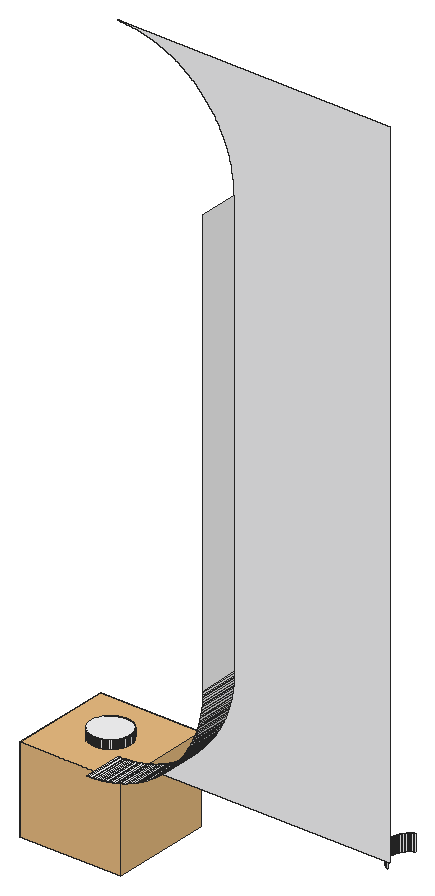
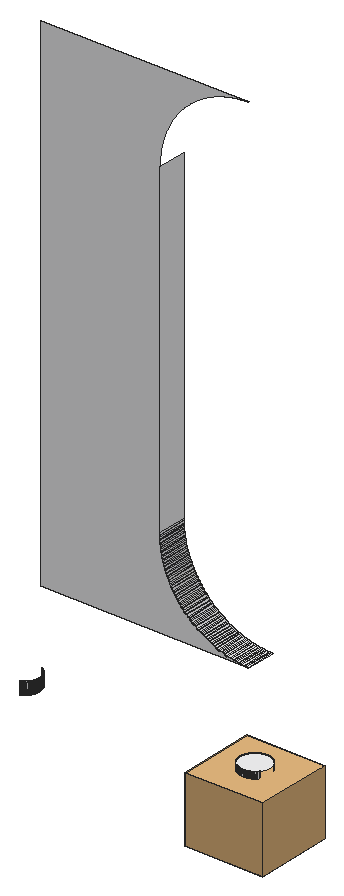
# SketchUp Ruby script. Lengths in inches.
U = 1.inch
M = Sketchup.active_model
def pt(a) = Geom::Point3d.new(a.map { |v| v * U })
def face(e, loops, mat)
  f = e.add_face(loops[0].map { |a| pt(a) })
  loops[1..].each { |l| e.add_face(l.map { |a| pt(a) }).erase! }
  f.material = f.back_material = mat if mat
  f
end
# faces: each face lists its corners as indices into pts; further lists are holes
def faces(e, pts, list, mat = nil) = list.each { |f| face(e, (f[0].is_a?(Array) ? f : [f]).map { |l| l.map { |i| pts[i] } }, mat) }
# xy, xz, yz: faces in a plane at the given z, y or x. An outline is a flat list of corners, or four numbers for a rectangle; further outlines are holes
def ring(l) = l.size == 4 ? [[l[0], l[1]], [l[2], l[1]], [l[2], l[3]], [l[0], l[3]]] : l.each_slice(2).to_a
def flat(e, list, mat, &to3) = list.each { |f| face(e, (f[0].is_a?(Array) ? f : [f]).map { |l| ring(l).map { |u, v| to3.(u, v) } }, mat) }
def xy(e, z, list, mat = nil) = flat(e, list, mat) { |x, y| [x, y, z] }
def xz(e, y, list, mat = nil) = flat(e, list, mat) { |x, z| [x, y, z] }
def yz(e, x, list, mat = nil) = flat(e, list, mat) { |y, z| [x, y, z] }
def lines(e, pts, list) = list.each { |a, b| e.add_line(pt(pts[a]), pt(pts[b])) }
# prism: a flat outline (further loops are holes) pulled along v
def prism(e, loops, v, mat = nil)
  f = face(e, loops, mat); d = Geom::Vector3d.new(v.map { |x| x * U })
  f.pushpull(f.normal.samedirection?(d) ? d.length : -d.length)
end
def box(e, o, s, mat = nil) = prism(e, [[o, [o[0] + s[0], o[1], o[2]], [o[0] + s[0], o[1] + s[1], o[2]], [o[0], o[1] + s[1], o[2]]]], [0, 0, s[2]], mat)
def at(x, y, z, deg = 0) = Geom::Transformation.translation(pt([x, y, z])) * Geom::Transformation.rotation(ORIGIN, Z_AXIS, deg.degrees)
def axes(o, x, y, z) = Geom::Transformation.new([*x, 0, *y, 0, *z, 0, *pt(o).to_a, 1])
def part(name) = M.definitions.add(name)
# library, detail: a bought-in or finely detailed component or shape, given as its bounding box
def library(name, o, s) = part(name).tap { |d| box(d.entities, o, s) }
def detail(e, o, s) = box(e.add_group.entities, o, s)
def put(e, d, t, mat = nil) = e.add_instance(d, t).tap { |i| i.material = mat if mat }
def group(e, t, mat = nil) = e.add_group.tap { |g| g.transformation = t; g.material = mat if mat }.entities
root = M.entities
M.materials.add("[Quartz Light Grey]").color = [251, 251, 252]
c1 = library("5",[-6.25,-6.25,-13.16],[15.58,15.58,13.16])
xy(root,119.5,[[161.51,204,161.35,204.02,161.28,204.03,161.12,204.05,161.04,204.07,160.97,204.08,160.89,204.1,160.81,204.125,160.74,204.15,160.67,204.17,160.59,204.2,160.45,204.26,160.375,204.29,160.3,204.33,160.24,204.36,160.03,204.48,159.97,204.53,159.9,204.57,159.6,204.82,159.55,204.88,159.49,204.93,159.4375,204.99,159.39,205.05,159.29,205.17,159.24,205.24,159.19,205.3,159.15,205.37,159.11,205.43,158.99,205.64,158.87,205.92,158.84,206,158.8125,206.07,158.79,206.15,158.77,206.22,158.75,206.3,158.73,206.375,158.72,206.45,158.7,206.53,158.69,206.61,158.68,206.6875,158.68,206.76,158.67,206.84,158.67,207.16,158.68,207.24,158.68,207.3125,158.69,207.39,158.7,207.47,158.72,207.55,158.73,207.625,158.75,207.7,158.77,207.78,158.79,207.85,158.8125,207.93,158.84,208,158.87,208.08,158.99,208.36,159.11,208.57,159.15,208.63,159.19,208.7,159.24,208.76,159.29,208.83,159.39,208.95,159.4375,209.01,159.49,209.07,159.55,209.12,159.6,209.18,159.9,209.43,159.97,209.47,160.03,209.52,160.24,209.64,160.3,209.67,160.375,209.71,160.45,209.74,160.59,209.8,160.67,209.83,160.74,209.85,160.81,209.875,160.89,209.9,160.97,209.92,161.04,209.93,161.12,209.95,161.28,209.97,161.35,209.98,161.51,210,161.82,210,162.14,209.96,162.21,209.95,162.29,209.93,162.37,209.92,162.44,209.9,162.52,209.875,162.59,209.85,162.67,209.83,162.81,209.77,162.89,209.74,162.96,209.71,163.03,209.67,163.1,209.64,163.17,209.6,163.23,209.56,163.3,209.52,163.37,209.47,163.43,209.43,163.55,209.33,163.62,209.28,163.67,209.23,163.73,209.18,163.9,209.01,164.05,208.83,164.09,208.76,164.14,208.7,164.18,208.63,164.22,208.57,164.34,208.36,164.41,208.22,164.4375,208.15,164.47,208.08,164.49,208,164.52,207.93,164.54,207.85,164.5625,207.78,164.58,207.7,164.62,207.55,164.64,207.39,164.65,207.3125,164.66,207.24,164.66,207.16,164.67,207.08,164.67,206.92,164.66,206.84,164.66,206.76,164.65,206.6875,164.64,206.61,164.62,206.45,164.58,206.3,164.5625,206.22,164.54,206.15,164.52,206.07,164.49,206,164.47,205.92,164.4375,205.85,164.41,205.78,164.34,205.64,164.22,205.43,164.18,205.37,164.14,205.3,164.09,205.24,164.05,205.17,163.9,204.99,163.73,204.82,163.67,204.77,163.62,204.72,163.55,204.67,163.43,204.57,163.37,204.53,163.3,204.48,163.23,204.44,163.17,204.4,163.1,204.36,163.03,204.33,162.96,204.29,162.89,204.26,162.81,204.23,162.67,204.17,162.59,204.15,162.52,204.125,162.44,204.1,162.37,204.08,162.29,204.07,162.21,204.05,162.14,204.04,161.82,204]],"[Quartz Light Grey]")
xy(root,126,[[174,187,174.24,193]],"[Quartz Light Grey]")
xy(root,126.01,[[174.47,187,174.71,193]],"[Quartz Light Grey]")
xz(root,193,[[174,126,174.24,126,174.47,126.01,174.71,126.01,174.94,126.02,175.18,126.04,175.41,126.06,175.65,126.08,175.88,126.1,176.12,126.125,176.35,126.15,176.58,126.1875,176.82,126.22,177.28,126.3,177.51,126.35,177.74,126.39,177.97,126.44,178.2,126.5,178.43,126.55,178.66,126.61,178.89,126.68,179.11,126.74,179.34,126.81,179.5625,126.88,179.79,126.96,180.01,127.03,180.23,127.11,180.45,127.2,180.67,127.28,181.11,127.46,181.32,127.56,181.54,127.65,181.75,127.75,181.96,127.86,182.17,127.96,182.59,128.18,182.8,128.3,183,128.41,183.4,128.65,183.61,128.78,183.8,128.9,184,129.03,184.2,129.17,184.39,129.3,184.58,129.4375,184.77,129.58,184.96,129.72,185.14,129.86,185.33,130.01,185.51,130.16,185.69,130.3125,185.87,130.47,186.04,130.625,186.22,130.78,186.39,130.94,186.56,131.11,186.73,131.27,186.89,131.44,187.06,131.61,187.22,131.78,187.375,131.96,187.53,132.13,187.6875,132.31,187.84,132.49,187.99,132.67,188.14,132.86,188.28,133.04,188.42,133.23,188.5625,133.42,188.7,133.61,188.83,133.8,188.97,134,189.1,134.2,189.22,134.39,189.35,134.6,189.59,135,189.7,135.2,189.82,135.41,190.04,135.83,190.14,136.04,190.25,136.25,190.35,136.46,190.44,136.68,190.54,136.89,190.72,137.33,190.8,137.55,190.89,137.77,190.97,137.99,191.04,138.21,191.12,138.4375,191.19,138.66,191.26,138.89,191.32,139.11,191.39,139.34,191.45,139.57,191.5,139.8,191.56,140.03,191.61,140.26,191.65,140.49,191.7,140.72,191.78,141.18,191.8125,141.42,191.85,141.65,191.875,141.88,191.9,142.12,191.92,142.35,191.94,142.59,191.96,142.82,191.98,143.06,191.99,143.29,191.99,143.53,192,143.76,192,210.24,191.99,210.47,191.99,210.71,191.98,210.94,191.96,211.18,191.94,211.41,191.92,211.65,191.9,211.88,191.875,212.12,191.85,212.35,191.8125,212.58,191.78,212.82,191.7,213.28,191.65,213.51,191.61,213.74,191.56,213.97,191.5,214.2,191.45,214.43,191.39,214.66,191.32,214.89,191.26,215.11,191.19,215.34,191.12,215.5625,191.04,215.79,190.97,216.01,190.89,216.23,190.8,216.45,190.72,216.67,190.54,217.11,190.44,217.32,190.35,217.54,190.25,217.75,190.14,217.96,190.04,218.17,189.82,218.59,189.7,218.8,189.59,219,189.35,219.4,189.22,219.61,189.1,219.8,188.97,220,188.83,220.2,188.7,220.39,188.5625,220.58,188.42,220.77,188.28,220.96,188.14,221.14,187.99,221.33,187.84,221.51,187.6875,221.69,187.53,221.87,187.375,222.04,187.22,222.22,187.06,222.39,186.89,222.56,186.73,222.73,186.56,222.89,186.39,223.06,186.22,223.22,186.04,223.375,185.87,223.53,185.69,223.6875,185.51,223.84,185.33,223.99,185.14,224.14,184.96,224.28,184.77,224.42,184.58,224.5625,184.39,224.7,184.2,224.83,184,224.97,183.8,225.1,183.61,225.22,183.4,225.35,183,225.59,182.8,225.7,182.59,225.82,182.17,226.04,181.96,226.14,181.75,226.25,181.54,226.35,181.32,226.44,181.11,226.54,180.67,226.72,180.45,226.8,180.23,226.89,180.01,226.97,179.79,227.04,179.5625,227.12,179.34,227.19,179.11,227.26,178.89,227.32,178.66,227.39,178.43,227.45,178.2,227.5,177.97,227.56,177.74,227.61,177.51,227.65,177.28,227.7,176.82,227.78,176.58,227.8125,176.35,227.85,176.12,227.875,175.88,227.9,175.65,227.92,175.41,227.94,175.18,227.96,174.94,227.98,174.71,227.99,174.47,227.99,174.24,228,174,228,216,228,216,126]],"[Quartz Light Grey]")
xz(root,204,[[161.51,117,161.59,119.5],[161.59,117,161.67,119.5],[161.67,117,161.75,119.5],[161.75,117,161.82,119.5]],"[Quartz Light Grey]")
xz(root,210,[[161.51,117,161.59,119.5],[161.59,117,161.67,119.5],[161.67,117,161.75,119.5],[161.75,117,161.82,119.5]],"[Quartz Light Grey]")
yz(root,164.66,[[206.76,117,206.84,119.5],[207.16,117,207.24,119.5]],"[Quartz Light Grey]")
yz(root,164.67,[[206.92,117,207,119.5],[207,117,207.08,119.5]],"[Quartz Light Grey]")
yz(root,191.99,[[187,143.29,193,143.53]],"[Quartz Light Grey]")
yz(root,192,[[187,143.76,193,144],[187,144,193,210]],"[Quartz Light Grey]")
yz(root,205,[[206.84,117,206.92,119.5],[206.92,117,207,119.5],[207,117,207.08,119.5],[207.08,117,207.16,119.5]],"[Quartz Light Grey]")
p = [[161.2,204.04,117],[161.12,204.05,117],[161.12,204.05,119.5],[161.2,204.04,119.5],[161.28,204.03,117],[161.28,204.03,119.5],
  [161.35,204.02,117],[161.35,204.02,119.5],[161.43,204.01,117],[161.43,204.01,119.5],[161.51,204,117],[161.51,204,119.5],
  [161.9,204.01,117],[161.82,204,117],[161.82,204,119.5],[161.9,204.01,119.5],[161.98,204.02,117],[161.98,204.02,119.5],
  [162.06,204.03,117],[162.06,204.03,119.5],[162.14,204.04,117],[162.14,204.04,119.5],[162.21,204.05,117],[162.21,204.05,119.5],
  [160.74,204.15,117],[160.67,204.17,117],[160.67,204.17,119.5],[160.74,204.15,119.5],[160.81,204.125,117],[160.81,204.125,119.5],
  [160.89,204.1,117],[160.89,204.1,119.5],[160.97,204.08,117],[160.97,204.08,119.5],[161.04,204.07,117],[161.04,204.07,119.5],
  [162.29,204.07,117],[162.29,204.07,119.5],[162.37,204.08,117],[162.37,204.08,119.5],[162.44,204.1,117],[162.44,204.1,119.5],
  [162.52,204.125,117],[162.52,204.125,119.5],[162.59,204.15,117],[162.59,204.15,119.5],[162.67,204.17,117],[162.67,204.17,119.5],
  [160.52,204.23,117],[160.45,204.26,117],[160.45,204.26,119.5],[160.52,204.23,119.5],[160.59,204.2,117],[160.59,204.2,119.5],
  [162.74,204.2,117],[162.74,204.2,119.5],[162.81,204.23,117],[162.81,204.23,119.5],[162.89,204.26,117],[162.89,204.26,119.5],
  [160.3,204.33,117],[160.24,204.36,117],[160.24,204.36,119.5],[160.3,204.33,119.5],[160.375,204.29,117],[160.375,204.29,119.5],
  [162.96,204.29,117],[162.96,204.29,119.5],[163.03,204.33,117],[163.03,204.33,119.5],[163.1,204.36,117],[163.1,204.36,119.5],
  [206.64,204.33,117],[206.57,204.36,117],[206.57,204.36,119.5],[206.64,204.33,119.5],[160.1,204.44,117],[160.03,204.48,117],
  [160.03,204.48,119.5],[160.1,204.44,119.5],[160.17,204.4,117],[160.17,204.4,119.5],[163.17,204.4,117],[163.17,204.4,119.5],
  [163.23,204.44,117],[163.23,204.44,119.5],[163.3,204.48,117],[163.3,204.48,119.5],[206.43,204.44,117],[206.37,204.48,117],
  [206.37,204.48,119.5],[206.43,204.44,119.5],[206.5,204.4,117],[206.5,204.4,119.5],[159.97,204.53,117],[159.9,204.57,117],
  [159.9,204.57,119.5],[159.97,204.53,119.5],[163.37,204.53,117],[163.37,204.53,119.5],[163.43,204.57,117],[163.43,204.57,119.5],
  [206.3,204.53,117],[206.24,204.57,117],[206.24,204.57,119.5],[206.3,204.53,119.5],[159.84,204.62,117],[159.78,204.67,117],
  [159.78,204.67,119.5],[159.84,204.62,119.5],[163.49,204.62,117],[163.49,204.62,119.5],[163.55,204.67,117],[163.55,204.67,119.5],
  [206.17,204.62,117],[206.11,204.67,117],[206.11,204.67,119.5],[206.17,204.62,119.5],[159.72,204.72,117],[159.66,204.77,117],
  [159.66,204.77,119.5],[159.72,204.72,119.5],[163.62,204.72,117],[163.62,204.72,119.5],[163.67,204.77,117],[163.67,204.77,119.5],
  [206.05,204.72,117],[205.99,204.77,117],[205.99,204.77,119.5],[206.05,204.72,119.5],[159.6,204.82,117],[159.55,204.88,117],
  [159.55,204.88,119.5],[159.6,204.82,119.5],[163.73,204.82,117],[163.73,204.82,119.5],[163.79,204.88,117],[163.79,204.88,119.5],
  [205.93,204.82,117],[205.88,204.88,117],[205.88,204.88,119.5],[205.93,204.82,119.5],[159.49,204.93,117],[159.4375,204.99,117],
  [159.4375,204.99,119.5],[159.49,204.93,119.5],[163.84,204.93,117],[163.84,204.93,119.5],[163.9,204.99,117],[163.9,204.99,119.5],
  [205.82,204.93,117],[205.77,204.99,117],[205.77,204.99,119.5],[205.82,204.93,119.5],[159.39,205.05,117],[159.39,205.05,119.5],
  [163.95,205.05,117],[163.95,205.05,119.5],[205.72,205.05,117],[205.72,205.05,119.5],[159.34,205.11,117],[159.34,205.11,119.5],
  [164,205.11,117],[164,205.11,119.5],[164.05,205.17,117],[164.05,205.17,119.5],[205.67,205.11,117],[205.62,205.17,117],
  [205.62,205.17,119.5],[205.67,205.11,119.5],[164.09,205.24,117],[164.09,205.24,119.5],[164.14,205.3,117],[164.14,205.3,119.5],
  [205.57,205.24,117],[205.53,205.3,117],[205.53,205.3,119.5],[205.57,205.24,119.5],[164.18,205.37,117],[164.18,205.37,119.5],
  [205.48,205.37,117],[205.48,205.37,119.5],[164.22,205.43,117],[164.22,205.43,119.5],[164.26,205.5,117],[164.26,205.5,119.5],
  [205.44,205.43,117],[205.4,205.5,117],[205.4,205.5,119.5],[205.44,205.43,119.5],[164.3,205.57,117],[164.3,205.57,119.5],
  [205.36,205.57,117],[205.36,205.57,119.5],[164.34,205.64,117],[164.34,205.64,119.5],[164.375,205.71,117],[164.375,205.71,119.5],
  [205.33,205.64,117],[205.29,205.71,117],[205.29,205.71,119.5],[205.33,205.64,119.5],[164.41,205.78,117],[164.41,205.78,119.5],
  [205.26,205.78,117],[205.26,205.78,119.5],[164.4375,205.85,117],[164.4375,205.85,119.5],[205.23,205.85,117],[205.23,205.85,119.5],
  [164.47,205.92,117],[164.47,205.92,119.5],[164.49,206,117],[164.49,206,119.5],[205.2,205.92,117],[205.17,206,117],
  [205.17,206,119.5],[205.2,205.92,119.5],[164.52,206.07,117],[164.52,206.07,119.5],[205.15,206.07,117],[205.15,206.07,119.5],
  [164.54,206.15,117],[164.54,206.15,119.5],[164.5625,206.22,117],[164.5625,206.22,119.5],[205.125,206.15,117],[205.1,206.22,117],
  [205.1,206.22,119.5],[205.125,206.15,119.5],[164.58,206.3,117],[164.58,206.3,119.5],[205.08,206.3,117],[205.08,206.3,119.5],
  [164.6,206.375,117],[164.6,206.375,119.5],[205.07,206.375,117],[205.07,206.375,119.5],[164.62,206.45,117],[164.62,206.45,119.5],
  [205.05,206.45,117],[205.05,206.45,119.5],[164.63,206.53,117],[164.63,206.53,119.5],[164.64,206.61,117],[164.64,206.61,119.5],
  [205.04,206.53,117],[205.03,206.61,117],[205.03,206.61,119.5],[205.04,206.53,119.5],[164.65,206.6875,117],[164.65,206.6875,119.5],
  [205.02,206.6875,117],[205.02,206.6875,119.5],[164.66,206.76,117],[164.66,206.76,119.5],[205.01,206.76,117],[205.01,206.76,119.5],
  [164.67,206.92,117],[164.66,206.84,117],[164.66,206.84,119.5],[164.67,206.92,119.5],[205,206.84,117],[205,206.84,119.5],
  [164.66,207.16,117],[164.67,207.08,117],[164.67,207.08,119.5],[164.66,207.16,119.5],[164.65,207.3125,117],[164.66,207.24,117],
  [164.66,207.24,119.5],[164.65,207.3125,119.5],[205,207.16,117],[205.01,207.24,117],[205.01,207.24,119.5],[205,207.16,119.5],
  [205.02,207.3125,117],[205.02,207.3125,119.5],[164.64,207.39,117],[164.64,207.39,119.5],[205.03,207.39,117],[205.03,207.39,119.5],
  [164.63,207.47,117],[164.63,207.47,119.5],[205.04,207.47,117],[205.04,207.47,119.5],[164.6,207.625,117],[164.62,207.55,117],
  [164.62,207.55,119.5],[164.6,207.625,119.5],[205.05,207.55,117],[205.05,207.55,119.5],[205.07,207.625,117],[205.07,207.625,119.5],
  [164.58,207.7,117],[164.58,207.7,119.5],[205.08,207.7,117],[205.08,207.7,119.5],[164.5625,207.78,117],[164.5625,207.78,119.5],
  [205.1,207.78,117],[205.1,207.78,119.5],[164.54,207.85,117],[164.54,207.85,119.5],[205.125,207.85,117],[205.125,207.85,119.5],
  [164.49,208,117],[164.52,207.93,117],[164.52,207.93,119.5],[164.49,208,119.5],[205.15,207.93,117],[205.15,207.93,119.5],
  [205.17,208,117],[205.17,208,119.5],[164.47,208.08,117],[164.47,208.08,119.5],[205.2,208.08,117],[205.2,208.08,119.5],
  [164.41,208.22,117],[164.4375,208.15,117],[164.4375,208.15,119.5],[164.41,208.22,119.5],[205.23,208.15,117],[205.23,208.15,119.5],
  [205.26,208.22,117],[205.26,208.22,119.5],[164.375,208.29,117],[164.375,208.29,119.5],[205.29,208.29,117],[205.29,208.29,119.5],
  [164.34,208.36,117],[164.34,208.36,119.5],[205.33,208.36,117],[205.33,208.36,119.5],[164.26,208.5,117],[164.3,208.43,117],
  [164.3,208.43,119.5],[164.26,208.5,119.5],[205.36,208.43,117],[205.36,208.43,119.5],[205.4,208.5,117],[205.4,208.5,119.5],
  [164.22,208.57,117],[164.22,208.57,119.5],[205.44,208.57,117],[205.44,208.57,119.5],[164.14,208.7,117],[164.18,208.63,117],
  [164.18,208.63,119.5],[164.14,208.7,119.5],[205.48,208.63,117],[205.48,208.63,119.5],[205.53,208.7,117],[205.53,208.7,119.5],
  [164.09,208.76,117],[164.09,208.76,119.5],[205.57,208.76,117],[205.57,208.76,119.5],[159.29,208.83,117],[159.34,208.89,117],
  [159.34,208.89,119.5],[159.29,208.83,119.5],[164,208.89,117],[164.05,208.83,117],[164.05,208.83,119.5],[164,208.89,119.5],
  [205.62,208.83,117],[205.62,208.83,119.5],[205.67,208.89,117],[205.67,208.89,119.5],[159.39,208.95,117],[159.39,208.95,119.5],
  [159.4375,209.01,117],[159.4375,209.01,119.5],[163.9,209.01,117],[163.95,208.95,117],[163.95,208.95,119.5],[163.9,209.01,119.5],
  [205.72,208.95,117],[205.72,208.95,119.5],[205.77,209.01,117],[205.77,209.01,119.5],[159.49,209.07,117],[159.49,209.07,119.5],
  [163.84,209.07,117],[163.84,209.07,119.5],[205.82,209.07,117],[205.82,209.07,119.5],[159.55,209.12,117],[159.55,209.12,119.5],
  [159.6,209.18,117],[159.6,209.18,119.5],[163.73,209.18,117],[163.79,209.12,117],[163.79,209.12,119.5],[163.73,209.18,119.5],
  [205.88,209.12,117],[205.88,209.12,119.5],[205.93,209.18,117],[205.93,209.18,119.5],[159.66,209.23,117],[159.66,209.23,119.5],
  [159.72,209.28,117],[159.72,209.28,119.5],[163.62,209.28,117],[163.67,209.23,117],[163.67,209.23,119.5],[163.62,209.28,119.5],
  [205.99,209.23,117],[205.99,209.23,119.5],[206.05,209.28,117],[206.05,209.28,119.5],[159.78,209.33,117],[159.78,209.33,119.5],
  [159.84,209.38,117],[159.84,209.38,119.5],[163.49,209.38,117],[163.55,209.33,117],[163.55,209.33,119.5],[163.49,209.38,119.5],
  [206.11,209.33,117],[206.11,209.33,119.5],[206.17,209.38,117],[206.17,209.38,119.5],[159.9,209.43,117],[159.9,209.43,119.5],
  [159.97,209.47,117],[159.97,209.47,119.5],[163.37,209.47,117],[163.43,209.43,117],[163.43,209.43,119.5],[163.37,209.47,119.5],
  [206.24,209.43,117],[206.24,209.43,119.5],[206.3,209.47,117],[206.3,209.47,119.5],[160.03,209.52,117],[160.03,209.52,119.5],
  [160.1,209.56,117],[160.1,209.56,119.5],[163.23,209.56,117],[163.3,209.52,117],[163.3,209.52,119.5],[163.23,209.56,119.5],
  [206.37,209.52,117],[206.37,209.52,119.5],[206.43,209.56,117],[206.43,209.56,119.5],[160.17,209.6,117],[160.17,209.6,119.5],
  [160.24,209.64,117],[160.24,209.64,119.5],[160.3,209.67,117],[160.3,209.67,119.5],[163.03,209.67,117],[163.1,209.64,117],
  [163.1,209.64,119.5],[163.03,209.67,119.5],[163.17,209.6,117],[163.17,209.6,119.5],[206.5,209.6,117],[206.5,209.6,119.5],
  [206.57,209.64,117],[206.57,209.64,119.5],[206.64,209.67,117],[206.64,209.67,119.5],[160.375,209.71,117],[160.375,209.71,119.5],
  [160.45,209.74,117],[160.45,209.74,119.5],[160.52,209.77,117],[160.52,209.77,119.5],[162.81,209.77,117],[162.89,209.74,117],
  [162.89,209.74,119.5],[162.81,209.77,119.5],[162.96,209.71,117],[162.96,209.71,119.5],[206.71,209.71,117],[206.71,209.71,119.5],
  [160.59,209.8,117],[160.59,209.8,119.5],[160.67,209.83,117],[160.67,209.83,119.5],[160.74,209.85,117],[160.74,209.85,119.5],
  [162.59,209.85,117],[162.67,209.83,117],[162.67,209.83,119.5],[162.59,209.85,119.5],[162.74,209.8,117],[162.74,209.8,119.5],
  [160.81,209.875,117],[160.81,209.875,119.5],[160.89,209.9,117],[160.89,209.9,119.5],[160.97,209.92,117],[160.97,209.92,119.5],
  [161.04,209.93,117],[161.04,209.93,119.5],[161.12,209.95,117],[161.12,209.95,119.5],[161.2,209.96,117],[161.2,209.96,119.5],
  [162.14,209.96,117],[162.21,209.95,117],[162.21,209.95,119.5],[162.14,209.96,119.5],[162.29,209.93,117],[162.29,209.93,119.5],
  [162.37,209.92,117],[162.37,209.92,119.5],[162.44,209.9,117],[162.44,209.9,119.5],[162.52,209.875,117],[162.52,209.875,119.5],
  [161.28,209.97,117],[161.28,209.97,119.5],[161.35,209.98,117],[161.35,209.98,119.5],[161.43,209.99,117],[161.43,209.99,119.5],
  [161.51,210,117],[161.51,210,119.5],[161.82,210,117],[161.9,209.99,117],[161.9,209.99,119.5],[161.82,210,119.5],
  [161.98,209.98,117],[161.98,209.98,119.5],[162.06,209.97,117],[162.06,209.97,119.5],[174.47,187,126.01],[174.47,193,126.01],
  [174.24,193,126],[174.24,187,126],[174.94,187,126.02],[174.94,193,126.02],[174.71,193,126.01],[174.71,187,126.01],
  [175.18,187,126.04],[175.18,193,126.04],[175.41,187,126.06],[175.41,193,126.06],[175.65,187,126.08],[175.65,193,126.08],
  [175.88,187,126.1],[175.88,193,126.1],[176.12,187,126.125],[176.12,193,126.125],[176.35,187,126.15],[176.35,193,126.15],
  [176.58,187,126.1875],[176.58,193,126.1875],[176.82,187,126.22],[176.82,193,126.22],[177.05,187,126.26],[177.05,193,126.26],
  [177.28,187,126.3],[177.28,193,126.3],[177.51,187,126.35],[177.51,193,126.35],[177.74,187,126.39],[177.74,193,126.39],
  [177.97,187,126.44],[177.97,193,126.44],[178.2,187,126.5],[178.2,193,126.5],[178.43,187,126.55],[178.43,193,126.55],
  [178.66,187,126.61],[178.66,193,126.61],[178.89,187,126.68],[178.89,193,126.68],[179.11,187,126.74],[179.11,193,126.74],
  [179.34,187,126.81],[179.34,193,126.81],[179.5625,187,126.88],[179.5625,193,126.88],[179.79,187,126.96],[179.79,193,126.96],
  [180.01,187,127.03],[180.01,193,127.03],[180.23,187,127.11],[180.23,193,127.11],[180.45,187,127.2],[180.45,193,127.2],
  [180.67,187,127.28],[180.67,193,127.28],[180.89,187,127.37],[180.89,193,127.37],[181.11,187,127.46],[181.11,193,127.46],
  [181.32,187,127.56],[181.32,193,127.56],[181.54,187,127.65],[181.54,193,127.65],[181.75,187,127.75],[181.75,193,127.75],
  [181.96,187,127.86],[181.96,193,127.86],[182.17,187,127.96],[182.17,193,127.96],[182.38,187,128.07],[182.38,193,128.07],
  [182.59,187,128.18],[182.59,193,128.18],[182.8,187,128.3],[182.8,193,128.3],[183,187,128.41],[183,193,128.41],
  [183.2,187,128.53],[183.2,193,128.53],[183.4,187,128.65],[183.4,193,128.65],[183.61,187,128.78],[183.61,193,128.78],
  [183.8,187,128.9],[183.8,193,128.9],[184,187,129.03],[184,193,129.03],[183.94,187,128.99],[184.2,187,129.17],
  [184.2,193,129.17],[184.39,187,129.3],[184.39,193,129.3],[184.58,187,129.4375],[184.58,193,129.4375],[184.77,187,129.58],
  [184.77,193,129.58],[184.96,187,129.72],[184.96,193,129.72],[185.14,187,129.86],[185.14,193,129.86],[185.33,187,130.01],
  [185.33,193,130.01],[185.51,187,130.16],[185.51,193,130.16],[185.69,187,130.3125],[185.69,193,130.3125],[185.87,187,130.47],
  [185.87,193,130.47],[186.04,187,130.625],[186.04,193,130.625],[186.22,187,130.78],[186.22,193,130.78],[186.39,187,130.94],
  [186.39,193,130.94],[186.56,187,131.11],[186.56,193,131.11],[186.73,187,131.27],[186.73,193,131.27],[186.89,187,131.44],
  [186.89,193,131.44],[187.06,187,131.61],[187.06,193,131.61],[187.22,187,131.78],[187.22,193,131.78],[187.375,187,131.96],
  [187.375,193,131.96],[187.53,187,132.13],[187.53,193,132.13],[187.6875,187,132.31],[187.6875,193,132.31],[187.84,187,132.49],
  [187.84,193,132.49],[187.99,187,132.67],[187.99,193,132.67],[188.14,187,132.86],[188.14,193,132.86],[188.28,187,133.04],
  [188.28,193,133.04],[188.42,187,133.23],[188.42,193,133.23],[188.5625,187,133.42],[188.5625,193,133.42],[188.7,187,133.61],
  [188.7,193,133.61],[188.83,187,133.8],[188.83,193,133.8],[188.97,187,134],[188.97,193,134],[189.1,187,134.2],
  [189.1,193,134.2],[189.22,187,134.39],[189.22,193,134.39],[189.35,187,134.6],[189.35,193,134.6],[189.47,187,134.8],
  [189.47,193,134.8],[189.59,187,135],[189.59,193,135],[189.7,187,135.2],[189.7,193,135.2],[189.82,187,135.41],
  [189.82,193,135.41],[189.93,187,135.62],[189.93,193,135.62],[190.04,187,135.83],[190.04,193,135.83],[190.14,187,136.04],
  [190.14,193,136.04],[190.25,187,136.25],[190.25,193,136.25],[190.35,187,136.46],[190.35,193,136.46],[190.44,187,136.68],
  [190.44,193,136.68],[190.54,187,136.89],[190.54,193,136.89],[190.63,187,137.11],[190.63,193,137.11],[190.72,187,137.33],
  [190.72,193,137.33],[190.8,187,137.55],[190.8,193,137.55],[190.89,187,137.77],[190.89,193,137.77],[190.97,187,137.99],
  [190.97,193,137.99],[191.04,187,138.21],[191.04,193,138.21],[191.12,187,138.4375],[191.12,193,138.4375],[191.19,187,138.66],
  [191.19,193,138.66],[191.26,187,138.89],[191.26,193,138.89],[191.32,187,139.11],[191.32,193,139.11],[191.39,187,139.34],
  [191.39,193,139.34],[191.45,187,139.57],[191.45,193,139.57],[191.5,187,139.8],[191.5,193,139.8],[191.56,187,140.03],
  [191.56,193,140.03],[191.61,187,140.26],[191.61,193,140.26],[191.65,187,140.49],[191.65,193,140.49],[191.7,187,140.72],
  [191.7,193,140.72],[191.74,187,140.95],[191.74,193,140.95],[191.78,187,141.18],[191.78,193,141.18],[191.8125,187,141.42],
  [191.8125,193,141.42],[191.85,187,141.65],[191.85,193,141.65],[191.875,187,141.88],[191.875,193,141.88],[191.9,187,142.12],
  [191.9,193,142.12],[191.92,187,142.35],[191.92,193,142.35],[191.94,187,142.59],[191.94,193,142.59],[191.96,187,142.82],
  [191.96,193,142.82],[191.98,187,143.06],[191.98,193,143.06],[191.99,187,143.29],[191.99,193,143.29],[192,187,143.76],
  [192,193,143.76],[191.99,193,143.53],[191.99,187,143.53],[183.97,187,128.99]]
faces(root,p,[[0,1,2,3],[4,0,3,5],[6,4,5,7],[8,6,7,9],[10,8,9,11],[12,13,14,15],[16,12,15,17],[18,16,17,19],
  [20,18,19,21],[22,20,21,23],[24,25,26,27],[28,24,27,29],[30,28,29,31],[32,30,31,33],[34,32,33,35],[1,34,35,2],
  [36,22,23,37],[38,36,37,39],[40,38,39,41],[42,40,41,43],[44,42,43,45],[46,44,45,47],[48,49,50,51],[52,48,51,53],
  [25,52,53,26],[54,46,47,55],[56,54,55,57],[58,56,57,59],[60,61,62,63],[64,60,63,65],[49,64,65,50],[66,58,59,67],
  [68,66,67,69],[70,68,69,71],[72,73,74,75],[76,77,78,79],[80,76,79,81],[61,80,81,62],[82,70,71,83],[84,82,83,85],
  [86,84,85,87],[88,89,90,91],[92,88,91,93],[73,92,93,74],[94,95,96,97],[77,94,97,78],[98,86,87,99],[100,98,99,101],
  [102,103,104,105],[89,102,105,90],[106,107,108,109],[95,106,109,96],[110,100,101,111],[112,110,111,113],[114,115,116,117],[103,114,117,104],
  [118,119,120,121],[107,118,121,108],[122,112,113,123],[124,122,123,125],[126,127,128,129],[115,126,129,116],[130,131,132,133],[119,130,133,120],
  [134,124,125,135],[136,134,135,137],[138,139,140,141],[127,138,141,128],[142,143,144,145],[131,142,145,132],[146,136,137,147],[148,146,147,149],
  [150,151,152,153],[139,150,153,140],[143,154,155,144],[156,148,149,157],[151,158,159,152],[154,160,161,155],[162,156,157,163],[164,162,163,165],
  [166,167,168,169],[158,166,169,159],[170,164,165,171],[172,170,171,173],[174,175,176,177],[167,174,177,168],[178,172,173,179],[175,180,181,176],
  [182,178,179,183],[184,182,183,185],[186,187,188,189],[180,186,189,181],[190,184,185,191],[187,192,193,188],[194,190,191,195],[196,194,195,197],
  [198,199,200,201],[192,198,201,193],[202,196,197,203],[199,204,205,200],[206,202,203,207],[204,208,209,205],[210,206,207,211],[212,210,211,213],
  [214,215,216,217],[208,214,217,209],[218,212,213,219],[215,220,221,216],[222,218,219,223],[224,222,223,225],[226,227,228,229],[220,226,229,221],
  [230,224,225,231],[227,232,233,228],[234,230,231,235],[232,236,237,233],[238,234,235,239],[236,240,241,237],[242,238,239,243],[244,242,243,245],
  [246,247,248,249],[240,246,249,241],[250,244,245,251],[247,252,253,248],[254,250,251,255],[252,256,257,253],[258,259,260,261],[256,262,263,257],
  [264,265,266,267],[268,269,270,271],[272,273,274,275],[273,276,277,274],[278,268,271,279],[276,280,281,277],[282,278,279,283],[280,284,285,281],
  [286,287,288,289],[287,282,283,288],[284,290,291,285],[290,292,293,291],[294,286,289,295],[292,296,297,293],[298,294,295,299],[296,300,301,297],
  [302,298,299,303],[300,304,305,301],[306,307,308,309],[307,302,303,308],[304,310,311,305],[310,312,313,311],[314,306,309,315],[312,316,317,313],
  [318,319,320,321],[319,314,315,320],[316,322,323,317],[322,324,325,323],[326,318,321,327],[324,328,329,325],[330,326,327,331],[328,332,333,329],
  [334,335,336,337],[335,330,331,336],[332,338,339,333],[338,340,341,339],[342,334,337,343],[340,344,345,341],[346,347,348,349],[347,342,343,348],
  [344,350,351,345],[350,352,353,351],[354,346,349,355],[352,356,357,353],[358,359,360,361],[362,363,364,365],[363,354,355,364],[356,366,367,357],
  [366,368,369,367],[359,370,371,360],[370,372,373,371],[374,375,376,377],[375,362,365,376],[368,378,379,369],[378,380,381,379],[372,382,383,373],
  [384,374,377,385],[380,386,387,381],[382,388,389,383],[388,390,391,389],[392,393,394,395],[393,384,385,394],[386,396,397,387],[396,398,399,397],
  [390,400,401,391],[400,402,403,401],[404,405,406,407],[405,392,395,406],[398,408,409,399],[408,410,411,409],[402,412,413,403],[412,414,415,413],
  [416,417,418,419],[417,404,407,418],[410,420,421,411],[420,422,423,421],[414,424,425,415],[424,426,427,425],[428,429,430,431],[429,416,419,430],
  [422,432,433,423],[432,434,435,433],[426,436,437,427],[436,438,439,437],[440,441,442,443],[441,428,431,442],[434,444,445,435],[444,446,447,445],
  [438,448,449,439],[448,450,451,449],[450,452,453,451],[454,455,456,457],[455,458,459,456],[458,440,443,459],[446,460,461,447],[460,462,463,461],
  [462,464,465,463],[452,466,467,453],[466,468,469,467],[468,470,471,469],[472,473,474,475],[473,476,477,474],[476,454,457,477],[464,478,479,465],
  [470,480,481,471],[480,482,483,481],[482,484,485,483],[486,487,488,489],[487,490,491,488],[490,472,475,491],[484,492,493,485],[492,494,495,493],
  [494,496,497,495],[496,498,499,497],[498,500,501,499],[500,502,503,501],[504,505,506,507],[505,508,509,506],[508,510,511,509],[510,512,513,511],
  [512,514,515,513],[514,486,489,515],[502,516,517,503],[516,518,519,517],[518,520,521,519],[520,522,523,521],[524,525,526,527],[525,528,529,526],
  [528,530,531,529],[530,504,507,531],[532,533,534,535],[536,537,538,539],[540,541,537,536],[542,543,541,540],[544,545,543,542],[546,547,545,544],
  [548,549,547,546],[550,551,549,548],[552,553,551,550],[554,555,553,552],[556,557,555,554],[558,559,557,556],[560,561,559,558],[562,563,561,560],
  [564,565,563,562],[566,567,565,564],[568,569,567,566],[570,571,569,568],[572,573,571,570],[574,575,573,572],[576,577,575,574],[578,579,577,576],
  [580,581,579,578],[582,583,581,580],[584,585,583,582],[586,587,585,584],[588,589,587,586],[590,591,589,588],[592,593,591,590],[594,595,593,592],
  [596,597,595,594],[598,599,597,596],[600,601,599,598],[602,603,601,600],[604,605,603,602],[606,607,605,604],[608,609,607,606],[610,611,609,608],
  [612,613,611,610],[614,615,613,612],[616,617,615,614],[618,619,617,616],[620,621,619,618,622],[623,624,621,620],[625,626,624,623],[627,628,626,625],
  [629,630,628,627],[631,632,630,629],[633,634,632,631],[635,636,634,633],[637,638,636,635],[639,640,638,637],[641,642,640,639],[643,644,642,641],
  [645,646,644,643],[647,648,646,645],[649,650,648,647],[651,652,650,649],[653,654,652,651],[655,656,654,653],[657,658,656,655],[659,660,658,657],
  [661,662,660,659],[663,664,662,661],[665,666,664,663],[667,668,666,665],[669,670,668,667],[671,672,670,669],[673,674,672,671],[675,676,674,673],
  [677,678,676,675],[679,680,678,677],[681,682,680,679],[683,684,682,681],[685,686,684,683],[687,688,686,685],[689,690,688,687],[691,692,690,689],
  [693,694,692,691],[695,696,694,693],[697,698,696,695],[699,700,698,697],[701,702,700,699],[703,704,702,701],[705,706,704,703],[707,708,706,705],
  [709,710,708,707],[711,712,710,709],[713,714,712,711],[715,716,714,713],[717,718,716,715],[719,720,718,717],[721,722,720,719],[723,724,722,721],
  [725,726,724,723],[727,728,726,725],[729,730,728,727],[731,732,730,729],[733,734,732,731],[735,736,734,733],[737,738,736,735],[739,740,738,737],
  [741,742,740,739],[743,744,742,741],[745,746,744,743],[747,748,746,745],[749,750,748,747],[751,752,750,749],[753,754,752,751],[755,756,754,753],
  [757,758,756,755],[759,760,758,757],[761,762,760,759],[763,764,762,761],[765,766,764,763],[767,768,769,770]],"[Quartz Light Grey]")
lines(root,p,[[622,771]])
put(root,c1,at(160.13,205.47,118.25),"[Quartz Light Grey]")
